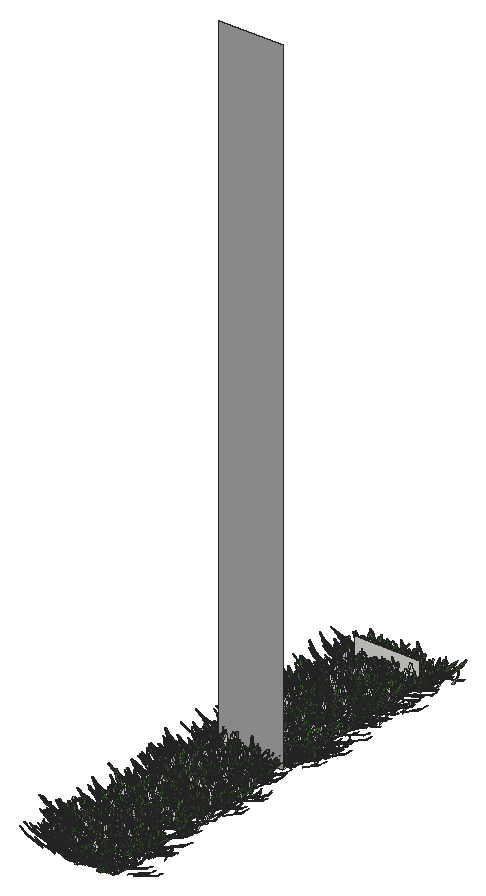
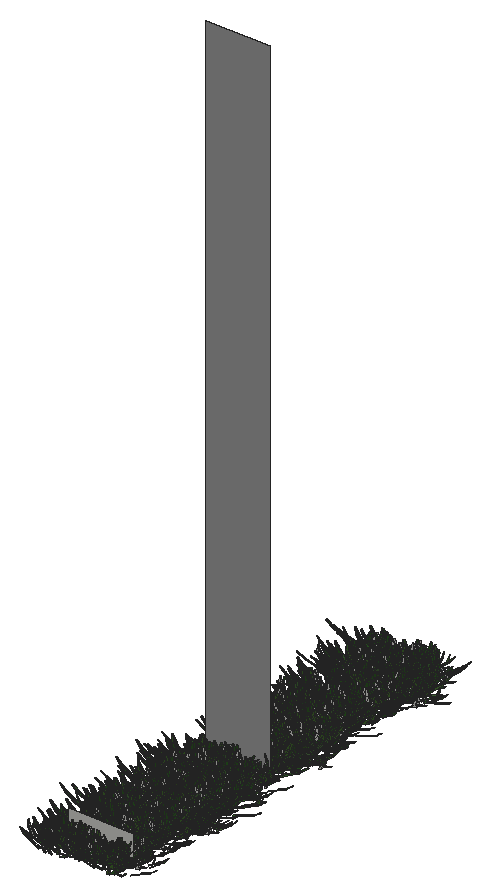
# SketchUp Ruby script. Lengths in inches.
U = 1.inch
M = Sketchup.active_model
def pt(a) = Geom::Point3d.new(a.map { |v| v * U })
def face(e, loops, mat)
  f = e.add_face(loops[0].map { |a| pt(a) })
  loops[1..].each { |l| e.add_face(l.map { |a| pt(a) }).erase! }
  f.material = f.back_material = mat if mat
  f
end
# faces: each face lists its corners as indices into pts; further lists are holes
def faces(e, pts, list, mat = nil) = list.each { |f| face(e, (f[0].is_a?(Array) ? f : [f]).map { |l| l.map { |i| pts[i] } }, mat) }
# xy, xz, yz: faces in a plane at the given z, y or x. An outline is a flat list of corners, or four numbers for a rectangle; further outlines are holes
def ring(l) = l.size == 4 ? [[l[0], l[1]], [l[2], l[1]], [l[2], l[3]], [l[0], l[3]]] : l.each_slice(2).to_a
def flat(e, list, mat, &to3) = list.each { |f| face(e, (f[0].is_a?(Array) ? f : [f]).map { |l| ring(l).map { |u, v| to3.(u, v) } }, mat) }
def xy(e, z, list, mat = nil) = flat(e, list, mat) { |x, y| [x, y, z] }
def xz(e, y, list, mat = nil) = flat(e, list, mat) { |x, z| [x, y, z] }
def yz(e, x, list, mat = nil) = flat(e, list, mat) { |y, z| [x, y, z] }
def lines(e, pts, list) = list.each { |a, b| e.add_line(pt(pts[a]), pt(pts[b])) }
# prism: a flat outline (further loops are holes) pulled along v
def prism(e, loops, v, mat = nil)
  f = face(e, loops, mat); d = Geom::Vector3d.new(v.map { |x| x * U })
  f.pushpull(f.normal.samedirection?(d) ? d.length : -d.length)
end
def box(e, o, s, mat = nil) = prism(e, [[o, [o[0] + s[0], o[1], o[2]], [o[0] + s[0], o[1] + s[1], o[2]], [o[0], o[1] + s[1], o[2]]]], [0, 0, s[2]], mat)
def at(x, y, z, deg = 0) = Geom::Transformation.translation(pt([x, y, z])) * Geom::Transformation.rotation(ORIGIN, Z_AXIS, deg.degrees)
def axes(o, x, y, z) = Geom::Transformation.new([*x, 0, *y, 0, *z, 0, *pt(o).to_a, 1])
def part(name) = M.definitions.add(name)
# library, detail: a bought-in or finely detailed component or shape, given as its bounding box
def library(name, o, s) = part(name).tap { |d| box(d.entities, o, s) }
def detail(e, o, s) = box(e.add_group.entities, o, s)
def put(e, d, t, mat = nil) = e.add_instance(d, t).tap { |i| i.material = mat if mat }
def group(e, t, mat = nil) = e.add_group.tap { |g| g.transformation = t; g.material = mat if mat }.entities
root = M.entities
M.materials.add("Material82").color = [68, 110, 58]
M.materials.add("Material83").color = [48, 90, 38]
M.materials.add("Material84").color = [68, 110, 48]
M.materials.add("Material85").color = [48, 90, 48]
M.materials.add("Material86").color = [58, 110, 58]
M.materials.add("Material87").color = [58, 90, 38]
M.materials.add("Material88").color = [68, 100, 58]
M.materials.add("Material89").color = [48, 100, 38]
M.materials.add("[Color M03]1").color = [170, 170, 170]
c1 = part("grass00")
p = [[-0.6875,0.15,0],[-0.56,0.08,5.52],[-0.04,0.03,2.76],[0.48,-0.02,0],[0.35,-0.02,5.52],[-0.1,-0.14,5.52],
  [-0.12,0.65,8.37],[-0.42,0.65,8.37]]
faces(c1.entities,p,[[0,1,2,3],[3,2,4],[1,5,2],[5,4,2],[1,6,5],[4,5,6],[7,6,1]])
c2 = part("Group16\#1")
put(c2.entities,c1,axes([1.44,-0.61,-0.01],[0.05352,0.12609,0],[-0.10704,0.04543,0.07239],[0.06664,-0.02828,0.11628]),"Material85")
put(c2.entities,c1,axes([0.76,-0.15,-0.01],[0.04676,0.24062,0],[-0.23162,0.04501,0.06642],[0.0652,-0.01267,0.23595]),"Material82")
put(c2.entities,c1,axes([0.79,0.01,-0.01],[-0.00606,0.34651,0],[-0.34381,-0.00602,0.0432],[0.04319,0.00076,0.34386]))
put(c2.entities,c1,axes([1,0.23,-0.01],[-0.07192,0.31144,0],[-0.28722,-0.06632,0.1236],[0.12043,0.02781,0.29478]),"Material84")
put(c2.entities,c1,axes([1.66,0.77,-0.01],[-0.13828,0.29651,0],[-0.21551,-0.1005,0.22471],[0.20365,0.09498,0.23779]),"Material89")
put(c2.entities,c1,axes([0.6875,0.52,-0.01],[-0.18126,0.24051,0],[-0.22746,-0.17142,0.09788],[0.07817,0.05891,0.28481]),"Material84")
put(c2.entities,c1,axes([0.68,0.78,-0.01],[-0.215,0.18688,0],[-0.12385,-0.14248,0.21334],[0.13995,0.16101,0.18878]),"Material82")
put(c2.entities,c1,axes([0.56,1,-0.01],[-0.13756,0.07624,0],[-0.06159,-0.11112,0.0927],[0.04494,0.08108,0.12705]),"Material84")
put(c2.entities,c1,axes([0.2,0.64,-0.01],[-0.23729,0.07254,0],[-0.05711,-0.18681,0.153],[0.04473,0.14632,0.19535]),"Material89")
put(c2.entities,c1,axes([0.0625,0.72,-0.01],[-0.28874,0.02525,0],[-0.02179,-0.24916,0.14647],[0.01276,0.14591,0.25012]),"Material82")
put(c2.entities,c1,axes([-0.08,0.62,-0.01],[-0.34089,-0.04187,0],[0.03255,-0.26504,0.216],[-0.02633,0.21439,0.26703]),"Material89")
put(c2.entities,c1,axes([-0.34,0.98,-0.01],[-0.14314,-0.0493,0],[0.04397,-0.12769,0.06843],[-0.02228,0.0647,0.13505]),"Material89")
put(c2.entities,c1,axes([-0.87,1.45,-0.01],[-0.23488,-0.14114,0],[0.13761,-0.22901,0.06087],[-0.03135,0.05217,0.26717]))
put(c2.entities,c1,axes([-0.72,0.77,-0.01],[-0.14208,-0.13251,0],[0.07209,-0.0773,0.16301],[-0.11118,0.11922,0.1057]),"Material89")
put(c2.entities,c1,axes([-0.62,0.43,-0.01],[-0.14845,-0.21203,0],[0.18654,-0.13061,0.12304],[-0.10079,0.07057,0.22772]),"Material82")
put(c2.entities,c1,axes([-0.68,0.29,-0.01],[-0.13639,-0.32136,0],[0.31723,-0.13464,0.05579],[-0.05136,0.0218,0.34462]),"Material83")
put(c2.entities,c1,axes([-0.64,0.125,-0.01],[-0.0458,-0.23569,0],[0.22124,-0.043,0.08276],[-0.08124,0.01579,0.22538]),"Material86")
put(c2.entities,c1,axes([-1.6,-0.03,-0.01],[0.00576,-0.32897,0],[0.27526,0.00482,0.18018],[-0.18015,-0.00315,0.2753]),"Material84")
put(c2.entities,c1,axes([-1.36,-0.31,-0.01],[0.05718,-0.24765,0],[0.18172,0.04196,0.17267],[-0.16825,-0.03885,0.1865]),"Material89")
put(c2.entities,c1,axes([-1.54,-0.72,-0.01],[0.06537,-0.14017,0],[0.13555,0.06321,0.03939],[-0.0357,-0.01665,0.14956]))
put(c2.entities,c1,axes([-1.19,-0.9,-0.01],[0.09597,-0.12735,0],[0.11214,0.08451,0.07557],[-0.06035,-0.04548,0.14042]),"Material88")
put(c2.entities,c1,axes([-0.47,-0.54,-0.01],[0.11588,-0.10072,0],[0.0618,0.0711,0.12124],[-0.07953,-0.0915,0.0942]))
put(c2.entities,c1,axes([-0.47,-0.84,-0.01],[0.11927,-0.0661,0],[0.06603,0.11913,0.00646],[-0.00313,-0.00565,0.13621]),"Material84")
put(c2.entities,c1,axes([-0.38,-1.24,-0.01],[0.28037,-0.08571,0],[0.0618,0.20215,0.20315],[-0.05939,-0.19428,0.21139]),"Material88")
put(c2.entities,c1,axes([-0.06,-0.66,-0.01],[0.22719,-0.01987,0],[0.01247,0.14255,0.17758],[-0.01547,-0.17691,0.1431]),"Material87")
put(c2.entities,c1,axes([0.11,-0.89,-0.01],[0.14882,0.01828,0],[-0.01058,0.08611,0.12229],[0.01491,-0.12138,0.08676]),"Material85")
put(c2.entities,c1,axes([0.25,-0.72,-0.01],[0.20481,0.07053,0],[-0.06206,0.18022,0.10291],[0.03351,-0.0973,0.1906]),"Material85")
put(c2.entities,c1,axes([0.85,-1.42,-0.01],[0.16481,0.09904,0],[-0.09472,0.15762,0.05616],[0.02893,-0.04814,0.18389]),"Material84")
put(c2.entities,c1,axes([1.01,-1.09,-0.01],[0.21858,0.20385,0],[-0.17495,0.1876,0.15339],[0.10462,-0.11218,0.25652]),"Material89")
put(c2.entities,c1,axes([1.01,-0.71,-0.01],[0.08733,0.12473,0],[-0.06445,0.04512,0.13037],[0.1068,-0.07477,0.07867]),"Material85")
c3 = part("Group15\#1")
put(c3.entities,c2,at(0,0,0))
c4 = part("3darcstudiotree_grass00\#1")
put(c4.entities,c3,at(0,0,0))
xy(root,-29.74,[[608.75,1000.12,626.34,1046.93]])
xz(root,1000.12,[[608.75,-29.74,626.34,149.375]],"[Color M03]1")
xz(root,1046.93,[[608.75,-29.74,626.34,-23.22]])
put(root,c4,axes([608.35,1026.73,-29.74],[3.58704,0.55594,0],[-1.39662,1.40151,-0.02634],[-0.05335,0.05353,1.58474]))
put(root,c4,axes([608.98,1011.3,-29.74],[3.13564,-0.95157,0],[2.13614,1.09478,-0.03629],[0.11919,0.06109,1.41389]))
put(root,c4,axes([608.58,989.93,-29.74],[2.62983,0.98737,0],[-2.70679,1.12128,-0.04733],[-0.14621,0.06057,1.31836]))
put(root,c4,axes([608.9375,952.45,-29.74],[2.45025,1.521,0],[-3.17244,0.79485,-0.05376],[-0.27331,0.06848,1.69687]))
put(root,c4,axes([609.1,1047.4,-29.74],[3.43516,0.20919,0],[-0.57575,1.47043,-0.03647],[-0.03089,0.0789,1.56991]))
put(root,c4,axes([609.01,955.45,-29.74],[3.99404,0.60234,0],[-1.558,1.60676,-0.01506],[-0.02517,0.02596,1.52965]))
put(root,c4,axes([610.85,1028.93,-29.74],[-3.8239,-0.32025,0],[0.87863,-1.63166,-0.02543],[0.02678,-0.04974,1.60712]))
put(root,c4,axes([610.86,948.67,-29.74],[-3.18903,-1.00454,0],[2.15912,-1.06605,-0.04095],[0.17363,-0.08573,1.76156]))
put(root,c4,axes([610.93,950.5,-29.74],[1.91072,-1.36379,0],[2.93743,0.64007,-0.00396],[0.02678,0.00583,1.94458]))
put(root,c4,axes([611.02,953.64,-29.74],[-3.96013,0.90558,0],[-1.84066,-1.25189,-0.01457],[-0.03554,-0.02417,1.33777]))
put(root,c4,axes([611.65,1023.41,-29.74],[-1.37854,-1.47975,0],[3.2131,-0.46555,-0.02344],[0.115,-0.01666,1.34096]))
put(root,c4,axes([611.49,1052.93,-29.74],[-3.78694,0.18795,0],[-0.43899,-1.37568,-0.01354],[-0.00909,-0.02849,1.41676]))
put(root,c4,axes([611.42,1005.67,-29.74],[-3.58928,0.33039,0],[-0.75882,-1.28211,-0.0198],[-0.02657,-0.04489,1.47686]))
put(root,c4,axes([611.25,1025.13,-29.74],[1.03001,-1.55898,0],[3.46185,0.35573,-0.04641],[0.24674,0.02535,1.47323]))
put(root,c4,axes([612,1020.6,-29.74],[0.07037,-1.71405,0],[4.70144,0.03002,-0.02796],[0.12644,0.00081,1.59394]))
put(root,c4,axes([611.23,981.91,-29.74],[-1.43633,1.59136,0],[-3.83282,-0.53804,-0.05045],[-0.25445,-0.03572,1.63245]))
put(root,c4,axes([612.67,961.375,-29.74],[-1.0696,-1.4156,0],[4.38412,-0.5152,-0.01047],[0.05162,-0.00607,1.7643]))
put(root,c4,axes([612.11,1018.05,-29.74],[-4.25189,0.62806,0],[-1.17044,-1.23238,-0.01358],[-0.02814,-0.02963,1.47772]))
put(root,c4,axes([610.86,983.55,-29.74],[1.80901,1.52238,0],[-3.47581,0.64237,-0.0367],[-0.2302,0.04254,1.99296]))
put(root,c4,axes([612.47,1016.5,-29.74],[-4.15804,-0.01553,0],[0.04454,-1.85443,-0.04475],[0.00172,-0.0718,1.43393]))
put(root,c4,axes([612.36,942.41,-29.74],[-3.28831,-0.06152,0],[0.17407,-1.44709,-0.03298],[0.01066,-0.08861,1.87797]))
put(root,c4,axes([612.51,992.37,-29.74],[-0.39059,-1.54022,0],[4.16557,-0.16429,-0.04439],[0.19629,-0.00774,1.39437]))
put(root,c4,axes([612.52,965.88,-29.74],[-3.41271,-0.33865,0],[0.85241,-1.336,-0.02412],[0.03639,-0.05703,1.61843]))
put(root,c4,axes([611.82,1032.22,-29.74],[2.99211,-0.88341,0],[2.54027,1.33816,-0.01707],[0.06311,0.03325,1.96039]))
put(root,c4,axes([612.67,1014.76,-29.74],[-3.68076,-0.30441,0],[0.87866,-1.65237,-0.00999],[0.00884,-0.01661,1.38276]))
put(root,c4,axes([611.35,1040.5,-29.74],[3.8777,-0.38352,0],[0.80355,1.2636,-0.03452],[0.06321,0.0994,1.86367]))
put(root,c4,axes([612.91,972.43,-29.74],[-2.93694,-0.59609,0],[2.12271,-1.62662,-0.00712],[0.01544,-0.01183,1.64666]))
put(root,c4,axes([612.39,974.29,-29.74],[-3.29904,0.80499,0],[-2.22234,-1.41651,-0.03047],[-0.07031,-0.04481,1.38852]))
put(root,c4,axes([611.74,990.88,-29.74],[4.14707,-0.51237,0],[1.30496,1.64274,-0.0458],[0.07431,0.09355,1.7756]))
put(root,c4,axes([612.3125,1028.2,-29.74],[-2.36198,1.34531,0],[-2.91809,-0.79683,-0.03104],[-0.17128,-0.04677,1.78553]))
put(root,c4,axes([611.42,945.82,-29.74],[3.27777,1.34463,0],[-2.52219,0.95624,-0.03508],[-0.15429,0.0585,1.59982]))
put(root,c4,axes([612.54,943.98,-29.74],[2.26051,-1.27757,0],[3.2134,0.8843,-0.05108],[0.25562,0.07035,1.79238]))
put(root,c4,axes([612.15,979.21,-29.74],[-1.59446,1.31407,0],[-3.90941,-0.73777,-0.03408],[-0.12847,-0.02424,1.35762]))
put(root,c4,axes([613.58,976.57,-29.74],[-0.30604,-1.61832,0],[4.50612,-0.13253,-0.02024],[0.10989,-0.00323,1.84439]))
put(root,c4,axes([612.78,1003.42,-29.74],[2.97125,-1.188,0],[2.63587,1.02532,-0.00165],[0.00768,0.00299,1.81884]))
put(root,c4,axes([612.76,968.1,-29.74],[3.41243,-1.19241,0],[2.8473,1.26731,-0.01442],[0.05672,0.02524,1.90876]))
put(root,c4,axes([612.42,963.68,-29.74],[-1.88838,1.28179,0],[-3.89061,-0.89146,-0.00809],[-0.03969,-0.00909,1.91363]))
put(root,c4,axes([612.06,1037.89,-29.74],[4.11116,0.47333,0],[-1.05643,1.42708,-0.03197],[-0.04362,0.05892,1.37583]))
put(root,c4,axes([613.02,994.52,-29.74],[2.99246,-1.30733,0],[3.43775,1.22386,-0.0538],[0.15792,0.05622,1.37259]))
put(root,c4,axes([613.94,1049.36,-29.74],[-3.25297,-0.61029,0],[1.91072,-1.58399,-0.03826],[0.09019,-0.07477,1.82966]))
put(root,c4,axes([613.82,998.96,-29.74],[-1.66901,-1.67644,0],[3.86369,-0.59826,-0.05278],[0.29329,-0.04541,1.85719]))
put(root,c4,axes([613.9375,1000.48,-29.74],[-4.35861,-0.14504,0],[0.36663,-1.71363,-0.02802],[0.01298,-0.06068,1.8014]))
put(root,c4,axes([612.83,958.125,-29.74],[3.20139,-0.30461,0],[0.92111,1.5056,-0.01591],[0.01676,0.0274,1.32206]))
put(root,c4,axes([612.63,1011.73,-29.74],[3.6615,0.00284,0],[-0.00662,1.32579,-0.0306],[-0.00046,0.09111,1.9022]))
put(root,c4,axes([614.16,987.83,-29.74],[0.73171,-1.70112,0],[4.49029,0.30039,-0.00997],[0.04273,0.00286,1.48373]))
put(root,c4,axes([614.04,1010.35,-29.74],[-3.40532,-0.07402,0],[0.22612,-1.61806,-0.00601],[0.00193,-0.01379,1.79325]))
put(root,c4,axes([614.125,1044.17,-29.74],[1.09339,-1.57965,0],[4.13626,0.44528,-0.00598],[0.02433,0.00262,1.35627]))
put(root,c4,axes([613.54,959.29,-29.74],[-2.68631,1.22242,0],[-2.89186,-0.98838,-0.03703],[-0.15503,-0.05299,1.58908]))
put(root,c4,axes([613.4,1043.42,-29.74],[3.3382,-1.0215,0],[2.0281,1.0308,-0.00126],[0.00417,0.00212,1.3431]))
put(root,c4,axes([612.77,985.51,-29.74],[1.0764,1.4346,0],[-4.21811,0.49224,-0.04809],[-0.1912,0.02231,1.36712]))
put(root,c4,axes([612.9,954.95,-29.74],[4.09217,0.10074,0],[-0.26997,1.70555,-0.00965],[-0.00291,0.01837,1.57035]))
put(root,c4,axes([613.77,1050.76,-29.74],[2.39,-1.25303,0],[3.55352,1.05416,-0.05537],[0.20037,0.05944,1.50911]))
put(root,c4,axes([613.24,1046.71,-29.74],[3.59653,-0.21085,0],[0.631,1.67397,-0.00967],[0.00626,0.01661,1.41667]))
put(root,c4,axes([613.04,997.02,-29.74],[1.32449,1.52251,0],[-4.11933,0.55735,-0.02597],[-0.14801,0.02003,1.96681]))
put(root,c4,axes([613.04,1008.23,-29.74],[3.15923,1.14894,0],[-3.00225,1.28393,-0.03053],[-0.12215,0.05224,1.95907]))
put(root,c4,axes([614.16,1036.36,-29.74],[-2.42169,0.94143,0],[-3.12641,-1.2508,-0.05994],[-0.19111,-0.07646,1.51606]))
put(root,c4,axes([613.32,1034.16,-29.74],[1.86247,1.54763,0],[-3.42195,0.64048,-0.01135],[-0.06523,0.01221,1.80626]))
put(root,c4,axes([614.34,971.02,-29.74],[3.3532,-0.49547,0],[1.21799,1.28203,-0.02122],[0.05381,0.05664,1.88089]))
put(root,c4,axes([616.32,983.625,-29.74],[-3.17181,-0.36437,0],[1.29907,-1.75875,-0.03129],[0.04635,-0.06275,1.8441]))
put(root,c4,axes([616.52,1034.68,-29.74],[-3.98386,-0.59662,0],[1.47731,-1.53422,-0.04397],[0.0965,-0.10022,1.92843]))
put(root,c4,axes([616.49,970.22,-29.74],[-3.51166,-0.15133,0],[0.49376,-1.78204,-0.01667],[0.00952,-0.03434,1.79039]))
put(root,c4,axes([616.08,1000.95,-29.74],[3.82244,-0.70635,0],[1.81239,1.52539,-0.00986],[0.01787,0.01504,1.36783]))
put(root,c4,axes([616.93,959.89,-29.74],[-4.25679,0.36903,0],[-0.81289,-1.45836,-0.01858],[-0.01888,-0.03387,1.34303]))
put(root,c4,axes([617.4,946.42,-29.74],[-2.72023,-1.01034,0],[2.91962,-1.22258,-0.03536],[0.13675,-0.05727,1.8008]))
put(root,c4,axes([616.53,1049.5,-29.74],[2.33818,-1.41789,0],[2.84176,0.72884,-0.04791],[0.27889,0.07153,1.76421]))
put(root,c4,axes([616.76,996.96,-29.74],[-2.05483,1.19866,0],[-3.00093,-0.80011,-0.04556],[-0.27207,-0.07254,1.95702]))
put(root,c4,axes([616.31,1035.5,-29.74],[3.87274,-0.73751,0],[1.55178,1.26734,-0.04306],[0.13654,0.11151,1.95064]))
put(root,c4,axes([617.04,1018.34,-29.74],[-3.50881,1.16011,0],[-2.69176,-1.26622,-0.04843],[-0.14054,-0.06611,1.41858]))
put(root,c4,axes([616.37,964.89,-29.74],[-0.97742,1.77445,0],[-3.78925,-0.32463,-0.03052],[-0.14263,-0.01222,1.38983]))
put(root,c4,axes([616.33,974.65,-29.74],[-0.8481,1.42544,0],[-3.97449,-0.36778,-0.03302],[-0.15824,-0.01464,1.5061]))
put(root,c4,axes([616.42,1012.76,-29.74],[3.5983,-0.42057,0],[0.96573,1.28508,-0.03127],[0.05191,0.06908,1.48816]))
put(root,c4,axes([616.43,1010.2,-29.74],[-1.39865,1.66077,0],[-3.78259,-0.49545,-0.00679],[-0.0282,-0.00369,1.30662]))
put(root,c4,axes([617.23,1023.18,-29.74],[2.65926,-1.384,0],[3.07673,0.91944,-0.04967],[0.23773,0.07104,1.73743]))
put(root,c4,axes([616.6,1040.71,-29.74],[3.19951,0.37191,0],[-1.24549,1.66647,-0.04213],[-0.05146,0.06886,1.42653]))
put(root,c4,axes([616.62,1005.14,-29.74],[3.23293,0.85538,0],[-2.19162,1.28829,-0.0468],[-0.14196,0.08345,1.60535]))
put(root,c4,axes([617.6875,945.21,-29.74],[1.73893,-1.7168,0],[3.5493,0.55914,-0.05078],[0.28442,0.04481,1.72798]))
put(root,c4,axes([616.88,942.34,-29.74],[1.27117,1.29221,0],[-3.51403,0.53763,-0.02781],[-0.14445,0.0221,1.57422]))
put(root,c4,axes([618.37,969.07,-29.74],[1.49045,-1.29572,0],[4.01852,0.71892,-0.00454],[0.01627,0.00291,1.30224]))
put(root,c4,axes([617.14,952.95,-29.74],[3.40006,0.04588,0],[-0.15479,1.78412,-0.02332],[-0.00425,0.049,1.80921]))
put(root,c4,axes([616.9,988.76,-29.74],[1.48796,1.33204,0],[-3.50735,0.60935,-0.02705],[-0.13278,0.02307,1.54111]))
put(root,c4,axes([617.33,1038.26,-29.74],[0.11998,1.39847,0],[-4.49149,0.05993,-0.06181],[-0.32467,0.00433,1.77032]))
put(root,c4,axes([618.34,1032.12,-29.74],[0.37423,-1.77165,0],[3.6892,0.1212,-0.04948],[0.31334,0.01029,1.76318]))
put(root,c4,axes([617.74,1029.67,-29.74],[-1.23102,1.43236,0],[-4.00109,-0.53481,-0.05878],[-0.24424,-0.03265,1.38915]))
put(root,c4,axes([619.01,1027.7,-29.74],[-3.85586,-0.61181,0],[1.38378,-1.3564,-0.02256],[0.04705,-0.04612,1.55256]))
put(root,c4,axes([617.53,1024.7,-29.74],[4.58666,-0.29954,0],[0.76961,1.83286,-0.06031],[0.05541,0.13196,1.9859]))
put(root,c4,axes([617.28,1044.86,-29.74],[3.04278,1.18912,0],[-3.29647,1.31191,-0.05903],[-0.21773,0.08665,1.83956]))
put(root,c4,axes([618.6,991.75,-29.74],[-3.4737,0.48099,0],[-1.22806,-1.37939,-0.01418],[-0.03068,-0.03446,1.8149]))
put(root,c4,axes([617.23,1015.74,-29.74],[2.59618,1.43862,0],[-2.87173,0.80602,-0.01154],[-0.04691,0.01317,1.31865]))
put(root,c4,axes([618.77,1003.42,-29.74],[0.50435,-1.60129,0],[3.80498,0.18639,-0.05019],[0.26525,0.01299,1.53052]))
put(root,c4,axes([617.38,981.16,-29.74],[1.0762,1.29593,0],[-3.71861,0.48029,-0.00037],[-0.00166,0.00021,1.37352]))
put(root,c4,axes([618.2,1050.99,-29.74],[-1.73323,1.28831,0],[-3.70175,-0.77456,-0.05129],[-0.19346,-0.04048,1.34106]))
put(root,c4,axes([619.08,962.09,-29.74],[-4.57816,0.34958,0],[-0.88534,-1.8033,-0.01839],[-0.0151,-0.03075,1.50803]))
put(root,c4,axes([619.32,950.24,-29.74],[-1.62742,-1.17488,0],[3.69115,-0.79521,-0.05959],[0.21649,-0.04664,1.30502]))
put(root,c4,axes([618.54,979.36,-29.74],[1.77469,-1.16148,0],[2.86416,0.68064,-0.04784],[0.28474,0.06767,1.7418]))
put(root,c4,axes([619.45,985.53,-29.74],[-0.38907,-1.30448,0],[3.64191,-0.16894,-0.01277],[0.06378,-0.00296,1.38207]))
put(root,c4,axes([618,977.57,-29.74],[0.22262,1.70783,0],[-4.21483,0.08545,-0.0387],[-0.20922,0.00424,1.71236]))
put(root,c4,axes([617.83,966.03,-29.74],[1.40686,1.47706,0],[-4.38712,0.6499,-0.05425],[-0.24934,0.03694,1.72469]))
put(root,c4,axes([618.25,995.02,-29.74],[3.74197,-0.40965,0],[1.02528,1.45661,-0.05393],[0.09104,0.12934,1.81331]))
put(root,c4,axes([618.06,1021.39,-29.74],[3.24935,0.42764,0],[-1.43334,1.69386,-0.04175],[-0.05922,0.06999,1.52086]))
put(root,c4,axes([619.93,1046.97,-29.74],[-3.23469,-1.08731,0],[2.23739,-1.03522,-0.02002],[0.06548,-0.0303,1.30322]))
put(root,c4,axes([618.43,1007.24,-29.74],[4.09406,-0.23131,0],[0.47213,1.29969,-0.032],[0.03631,0.09996,1.99674]))
put(root,c4,axes([618.77,948.56,-29.74],[-1.63246,1.63511,0],[-3.4831,-0.54085,-0.00571],[-0.03452,-0.00536,1.8245]))
put(root,c4,axes([618.98,958.01,-29.74],[-0.95146,1.7451,0],[-3.70497,-0.31417,-0.03186],[-0.21482,-0.01822,1.95913]))
put(root,c4,axes([618.86,999.34,-29.74],[1.78223,1.25772,0],[-3.10123,0.68348,-0.02391],[-0.11693,0.02577,1.49173]))
put(root,c4,axes([618.87,1014.125,-29.74],[0.65139,1.7147,0],[-4.45072,0.26296,-0.01905],[-0.08769,0.00518,1.57029]))
put(root,c4,axes([620.02,990.52,-29.74],[3.26505,-0.4107,0],[1.3901,1.71877,-0.05774],[0.0978,0.12093,1.91123]))
put(root,c4,axes([619.64,1042.77,-29.74],[4.04452,0.28903,0],[-0.72611,1.58031,-0.0513],[-0.04641,0.10101,1.54883]))
put(root,c4,axes([619.86,973.51,-29.74],[2.80643,0.90661,0],[-2.10951,1.0156,-0.00694],[-0.02809,0.01352,1.5947]))
put(root,c4,axes([620.08,956.04,-29.74],[4.57178,0.1006,0],[-0.19659,1.38952,-0.03032],[-0.00983,0.06951,1.54015]))
put(root,c4,axes([621.77,990.43,-29.74],[-3.18088,-0.40858,0],[1.35408,-1.63957,-0.00123],[0.00227,-0.00275,1.95221]))
put(root,c4,axes([622.15,1029.98,-29.74],[-3.04991,-1.12114,0],[2.90905,-1.23081,-0.00052],[0.00199,-0.00084,1.79691]))
put(root,c4,axes([622.59,955.34,-29.74],[-2.17426,-1.31341,0],[3.93463,-1.01304,-0.04707],[0.15585,-0.04013,1.39282]))
put(root,c4,axes([622.16,1049.56,-29.74],[0.86182,-1.33711,0],[3.4036,0.34119,-0.00558],[0.03445,0.00345,1.6757]))
put(root,c4,axes([622.08,1042.06,-29.74],[1.86264,-1.28665,0],[3.53883,0.79678,-0.00497],[0.01917,0.00432,1.35772]))
put(root,c4,axes([622.24,946.54,-29.74],[-3.35474,0.10257,0],[-0.29043,-1.4774,-0.03359],[-0.01806,-0.09187,1.95875]))
put(root,c4,axes([621.875,977.25,-29.74],[3.26089,-0.9276,0],[2.41726,1.32164,-0.00659],[0.02436,0.01332,1.95827]))
put(root,c4,axes([621.67,942.91,-29.74],[3.92346,-0.38379,0],[1.02863,1.63546,-0.04456],[0.04806,0.07641,1.43455]))
put(root,c4,axes([622.375,1045.63,-29.74],[2.18615,-1.3842,0],[3.44906,0.84721,-0.04551],[0.21226,0.05214,1.67334]))
put(root,c4,axes([623.34,972.5,-29.74],[-3.24318,-0.61658,0],[1.47082,-1.20323,-0.00927],[0.0316,-0.02585,1.99366]))
put(root,c4,axes([622.17,1032.54,-29.74],[2.25035,1.16277,0],[-2.68664,0.80868,-0.04536],[-0.27393,0.08245,1.92466]))
put(root,c4,axes([623.89,952.86,-29.74],[-0.91872,-1.28532,0],[4.49567,-0.49978,-0.01485],[0.07367,-0.00819,1.80381]))
put(root,c4,axes([623.18,966.19,-29.74],[0.6017,-1.37989,0],[3.88457,0.26344,-0.05034],[0.29768,0.02019,1.77282]))
put(root,c4,axes([622.53,944.49,-29.74],[3.93415,-0.89756,0],[1.9948,1.35987,-0.042],[0.11006,0.07503,1.56273]))
put(root,c4,axes([622.71,994.13,-29.74],[-1.11116,1.30676,0],[-3.31516,-0.43843,-0.03292],[-0.23061,-0.0305,1.93659]))
put(root,c4,axes([622.48,1051.8,-29.74],[-1.19077,1.57344,0],[-3.27951,-0.38601,-0.00408],[-0.02113,-0.00249,1.38631]))
put(root,c4,axes([623.625,1034.52,-29.74],[-0.12471,-1.80139,0],[4.72201,-0.05084,-0.06757],[0.3331,-0.00359,1.74608]))
put(root,c4,axes([623.8,1027.62,-29.74],[0.23876,-1.55199,0],[4.36064,0.10434,-0.04584],[0.18368,0.0044,1.3146]))
put(root,c4,axes([624.07,1010.22,-29.74],[-0.00481,-1.55543,0],[4.64446,-0.00224,-0.02113],[0.08601,-0.00004,1.41674]))
put(root,c4,axes([622.73,1003.14,-29.74],[3.47227,-0.30693,0],[0.74979,1.31925,-0.01015],[0.01336,0.0235,1.54623]))
put(root,c4,axes([622.7,1005.14,-29.74],[-1.26342,1.38148,0],[-3.54227,-0.50384,-0.00809],[-0.04856,-0.00691,1.80065]))
put(root,c4,axes([624.28,1053.54,-29.74],[-2.41696,-1.08887,0],[3.39352,-1.17154,-0.03006],[0.11594,-0.04003,1.73276]))
put(root,c4,axes([623.34,1011.81,-29.74],[2.94151,-0.90679,0],[2.69176,1.35804,-0.00613],[0.02014,0.01016,1.74641]))
put(root,c4,axes([622.61,1024.44,-29.74],[0.11831,1.37685,0],[-3.50344,0.04682,-0.00216],[-0.01444,0.00019,1.758]))
put(root,c4,axes([624.05,979.07,-29.74],[-1.52685,-1.32373,0],[3.20025,-0.57411,-0.03768],[0.23061,-0.04137,1.77164]))
put(root,c4,axes([623.15,984.47,-29.74],[-1.03634,1.43503,0],[-4.07668,-0.45789,-0.05457],[-0.22787,-0.02559,1.37935]))
put(root,c4,axes([623.97,1047.4,-29.74],[0.26998,-1.38938,0],[4.08981,0.1236,-0.05496],[0.34231,0.01035,1.9204]))
put(root,c4,axes([624.26,1015.1,-29.74],[-0.73982,-1.44093,0],[3.74487,-0.29904,-0.04711],[0.2431,-0.01941,1.50792]))
put(root,c4,axes([623.43,1036.5625,-29.74],[3.32502,-0.81851,0],[2.11953,1.33913,-0.03499],[0.11667,0.07371,1.88939]))
put(root,c4,axes([623.75,1020.44,-29.74],[2.48182,-1.04217,0],[2.75852,1.02169,-0.02466],[0.10108,0.03744,1.59511]))
put(root,c4,axes([623.59,1007.79,-29.74],[-2.81085,1.01922,0],[-2.91901,-1.25203,-0.0061],[-0.02341,-0.01004,1.83281]))
put(root,c4,axes([624.4,985.96,-29.74],[-3.57412,-0.0033,0],[0.00935,-1.57631,-0.04252],[0.00057,-0.09613,1.71753]))
